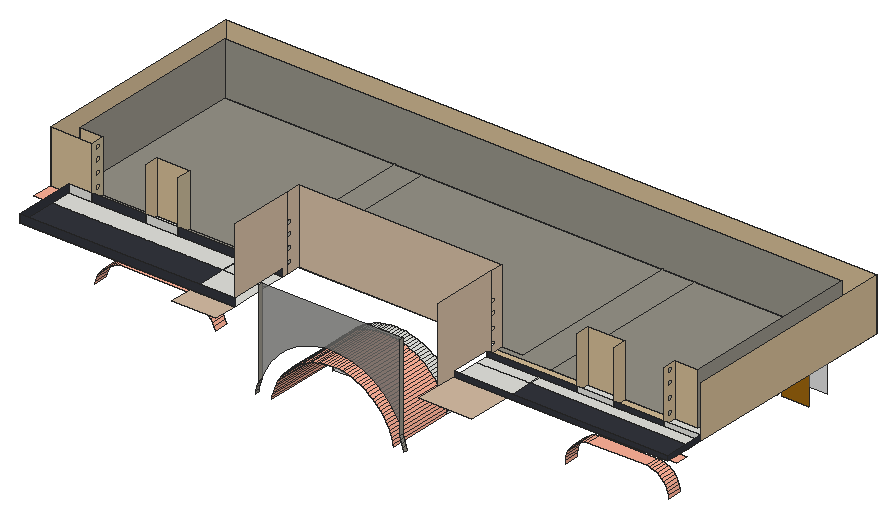
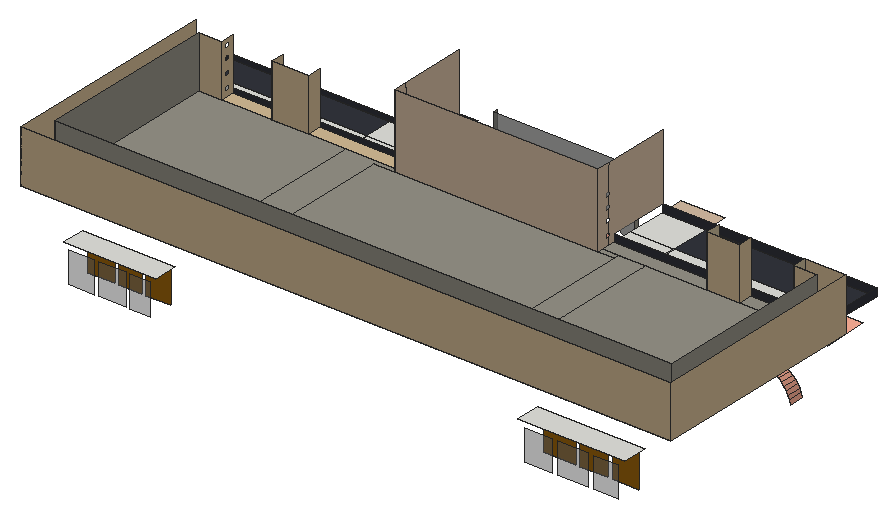
# SketchUp Ruby script. Lengths in inches.
U = 1.inch
M = Sketchup.active_model
def pt(a) = Geom::Point3d.new(a.map { |v| v * U })
def face(e, loops, mat)
  f = e.add_face(loops[0].map { |a| pt(a) })
  loops[1..].each { |l| e.add_face(l.map { |a| pt(a) }).erase! }
  f.material = f.back_material = mat if mat
  f
end
# faces: each face lists its corners as indices into pts; further lists are holes
def faces(e, pts, list, mat = nil) = list.each { |f| face(e, (f[0].is_a?(Array) ? f : [f]).map { |l| l.map { |i| pts[i] } }, mat) }
# xy, xz, yz: faces in a plane at the given z, y or x. An outline is a flat list of corners, or four numbers for a rectangle; further outlines are holes
def ring(l) = l.size == 4 ? [[l[0], l[1]], [l[2], l[1]], [l[2], l[3]], [l[0], l[3]]] : l.each_slice(2).to_a
def flat(e, list, mat, &to3) = list.each { |f| face(e, (f[0].is_a?(Array) ? f : [f]).map { |l| ring(l).map { |u, v| to3.(u, v) } }, mat) }
def xy(e, z, list, mat = nil) = flat(e, list, mat) { |x, y| [x, y, z] }
def xz(e, y, list, mat = nil) = flat(e, list, mat) { |x, z| [x, y, z] }
def yz(e, x, list, mat = nil) = flat(e, list, mat) { |y, z| [x, y, z] }
def lines(e, pts, list) = list.each { |a, b| e.add_line(pt(pts[a]), pt(pts[b])) }
# prism: a flat outline (further loops are holes) pulled along v
def prism(e, loops, v, mat = nil)
  f = face(e, loops, mat); d = Geom::Vector3d.new(v.map { |x| x * U })
  f.pushpull(f.normal.samedirection?(d) ? d.length : -d.length)
end
def box(e, o, s, mat = nil) = prism(e, [[o, [o[0] + s[0], o[1], o[2]], [o[0] + s[0], o[1] + s[1], o[2]], [o[0], o[1] + s[1], o[2]]]], [0, 0, s[2]], mat)
def at(x, y, z, deg = 0) = Geom::Transformation.translation(pt([x, y, z])) * Geom::Transformation.rotation(ORIGIN, Z_AXIS, deg.degrees)
def axes(o, x, y, z) = Geom::Transformation.new([*x, 0, *y, 0, *z, 0, *pt(o).to_a, 1])
def part(name) = M.definitions.add(name)
# library, detail: a bought-in or finely detailed component or shape, given as its bounding box
def library(name, o, s) = part(name).tap { |d| box(d.entities, o, s) }
def detail(e, o, s) = box(e.add_group.entities, o, s)
def put(e, d, t, mat = nil) = e.add_instance(d, t).tap { |i| i.material = mat if mat }
def group(e, t, mat = nil) = e.add_group.tap { |g| g.transformation = t; g.material = mat if mat }.entities
root = M.entities
M.materials.add("[Blinds Wood Light]").color = [155, 100, 14]
M.materials.add("[Color B02]").color = [255, 178, 153]
M.materials.add("[Formica Beige]").color = [211, 187, 149]
M.materials.add("[Formica Graystone]").color = [149, 146, 135]
M.materials.add("[Formica Laminate Dark]").color = [50, 53, 60]
M.materials.add("[Formica Laminate Light]").color = [213, 189, 164]
M.materials.add("[Quartz Light Brown]").color = [199, 184, 152]
M.materials.add("[Translucent Glass Block Dark]").color = [124, 124, 121]
M.materials["[Translucent Glass Block Dark]"].alpha = 0.8
M.materials.add("[Translucent Glass Gray]").color = [128, 128, 128]
M.materials["[Translucent Glass Gray]"].alpha = 0.5
M.materials.add("[Wood Veneer 01]3").color = [84, 49, 25]
xy(root,232.71,[[59.64,451.42,100.125,459.89]],"[Color B02]")
xy(root,236.125,[[341.29,451.42,376.4,459.89]],"[Color B02]")
xy(root,239.54,[[327.9375,568.57,383.25,583.14]])
xy(root,240.46,[[45.27,568.57,109.65,583.14]])
xy(root,249.06,[[311.91,444.11,400.54,451.42]],"[Color B02]")
xy(root,250.57,[[28.78,438.8,131.42,451.42]],"[Color B02]")
xy(root,261,[[131.42,414.84,157.59,438.8],[280.13,426.61,311.91,444.11],[28.78,438.8,131.42,451.42],[131.42,438.8,157.59,451.42],[280.13,444.11,311.91,451.42],
  [311.91,444.11,409.38,451.42],[17.625,451.42,17.625,583.14,409.38,583.14,409.38,451.42,386.6,451.42,386.6,459.89,400.54,459.89,400.54,568.57,28.78,568.57,28.78,459.89,42.4,459.89,42.4,451.42],[74.87,451.42,94.58,459.89],[334.34,451.42,356.76,459.89]])
xy(root,261,[[17.625,438.8,28.78,451.42]],"[Color B02]")
xy(root,261,[[280.13,451.42,334.34,459.89],[356.76,451.42,386.6,459.89]],"[Formica Beige]")
xy(root,261,[[42.4,451.42,74.87,459.89],[94.58,451.42,157.59,459.89],[28.78,459.89,131.42,568.57],[131.42,459.89,147.71,568.57],[147.71,459.89,157.59,463.02],
  [280.13,459.89,311.91,459.89,311.91,568.57,292.81,568.57,292.81,463.02,280.13,463.02],[311.91,459.89,400.54,568.57],[147.71,463.02,292.81,568.57]],"[Formica Graystone]")
xy(root,261,[[28.78,414.84,131.42,438.8],[311.91,426.61,409.38,444.11]],"[Formica Laminate Dark]")
xy(root,261,[[131.42,400.56,157.59,414.84],[280.13,400.56,311.91,426.61]],"[Formica Laminate Light]")
xz(root,414.84,[[28.78,261,157.59,265.6875]],"[Formica Laminate Dark]")
xz(root,414.84,[[174.14,227.22,174.4,227.97,175.18,229.93,176.05,231.85,177.02,233.73,178.07,235.57,179.2,237.35,180.42,239.08,181.71,240.75,183.08,242.36,184.53,243.9,186.04,245.375,187.63,246.77,189.27,248.1,190.98,249.34,192.74,250.51,194.56,251.59,196.42,252.59,198.33,253.49,200.28,254.3125,202.27,255.04,204.28,255.67,206.33,256.21,208.39,256.65,210.48,256.99,212.58,257.24,214.6875,257.39,216.8,257.44,218.91,257.39,221.02,257.24,223.12,256.99,225.21,256.65,227.27,256.21,229.32,255.67,231.33,255.04,233.32,254.3125,235.27,253.49,237.18,252.59,239.04,251.59,240.86,250.51,242.62,249.34,244.33,248.1,245.97,246.77,247.56,245.375,249.07,243.9,250.52,242.36,251.89,240.75,253.18,239.08,254.4,237.35,255.53,235.57,256.58,233.73,257.55,231.85,258.42,229.93,259.2,227.97,259.2,279.69,174.14,279.69]],"[Translucent Glass Block Dark]")
xz(root,426.61,[[280.13,261,409.38,263.9375]],"[Formica Laminate Dark]")
xz(root,451.42,[[28.78,261,42.4,265.6875],[74.87,261,94.58,265.6875],[334.34,261,356.76,263.9375],[386.6,261,409.38,263.9375]])
xz(root,451.42,[[17.625,261,28.78,261,28.78,265.6875,42.4,265.6875,42.4,292.375,17.625,292.375]],"[Formica Beige]")
xz(root,451.42,[[42.4,261,74.87,265.6875],[94.58,261,157.59,265.6875],[280.13,261,334.34,263.9375],[356.76,261,386.6,263.9375]],"[Formica Laminate Dark]")
xz(root,454.92,[[185.03,218.57,185.14,219.14,185.03,219.14],[248.46,218.57,248.57,218.57,248.46,219.14]])
xz(root,454.92,[[185.03,218.57,199.57,218.57,199.57,239.64,198.3,238.81,197.08,237.91,195.9,236.97,194.77,235.96,193.68,234.91,192.65,233.8,191.66,232.65,190.74,231.46,189.86,230.22,189.05,228.9375,188.3,227.625,187.61,226.28,186.99,224.9,186.42,223.49,185.93,222.0625,185.5,220.61,185.14,219.14],[202.18,218.57,213.78,218.57,213.78,244.46,212.27,244.29,210.78,244.04,209.3,243.72,207.83,243.34,206.39,242.89,204.97,242.37,203.57,241.78,202.2,241.13],[218.3125,218.57,233.875,218.57,234.03,239.64,232.73,240.42,231.4,241.13,230.03,241.78,228.63,242.37,227.21,242.89,225.77,243.34,224.3,243.72,222.82,244.04,221.33,244.29,219.82,244.46,218.3125,244.57],[236.52,218.57,248.46,218.57,248.46,219.14,248.1,220.61,247.67,222.0625,247.17,223.49,246.61,224.9,245.99,226.28,245.3,227.625,244.55,228.9375,243.73,230.22,242.86,231.46,241.9375,232.65,240.95,233.8,239.92,234.91,238.83,235.96,237.7,236.97,236.52,237.91]],"[Translucent Glass Gray]")
xz(root,454.92,[[199.57,218.57,202.18,218.57,202.2,241.13,200.87,240.42,199.57,239.64],[213.78,218.57,218.3125,218.57,218.3125,244.57,216.8,244.6,215.29,244.57,213.78,244.46],[233.875,218.57,236.52,218.57,236.52,237.91,235.3,238.81,234.03,239.64]],"[Wood Veneer 01]3")
xz(root,459.89,[[28.78,261,42.4,292.375],[74.87,261,94.58,292.375],[334.34,261,356.76,292.375],[386.6,261,400.54,292.375]],"[Formica Beige]")
xz(root,463.02,[[157.59,261,280.13,305.4375]],"[Formica Laminate Light]")
xz(root,568.57,[[48.75,217.42,64.6,236.99],[67.24,217.42,84.0625,236.99],[86.71,217.42,106.17,236.99],[330.49,217.74,345.72,236.98],[348.05,217.74,362.04,236.98],
  [364.37,217.74,380.69,236.98]],"[Blinds Wood Light]")
xz(root,568.57,[[28.78,261,400.54,292.375]],"[Formica Graystone]")
xz(root,583.14,[[17.625,261,409.38,292.375]],"[Formica Beige]")
xz(root,583.14,[[330.83,217.46,343.23,236.65],[345.56,217.46,362.04,236.65],[364.37,217.46,380.36,236.65],[49,218.21,64.12,236.74],[67.33,218.21,85.93,236.74],
  [89.14,218.21,105.92,236.74]],"[Translucent Glass Gray]")
yz(root,17.625,[[451.42,261,583.14,292.375]],"[Formica Beige]")
yz(root,28.78,[[459.89,261,568.57,292.375]],"[Formica Graystone]")
yz(root,28.78,[[414.84,261,451.42,265.6875]],"[Formica Laminate Dark]")
yz(root,42.4,[[[451.42,261,459.89,292.375],[456.03,265.2,455.63,265.25,455.25,265.41,454.93,265.66,454.68,265.98,454.52,266.36,454.47,266.76,454.52,267.17,454.68,267.54,454.93,267.87,455.25,268.11,455.63,268.27,456.03,268.32,456.4375,268.27,456.8125,268.11,457.14,267.87,457.39,267.54,457.54,267.17,457.6,266.76,457.54,266.36,457.39,265.98,457.14,265.66,456.8125,265.41,456.4375,265.25],[456.03,280.26,455.63,280.3125,455.25,280.47,454.93,280.72,454.68,281.04,454.52,281.42,454.47,281.82,454.52,282.23,454.68,282.6,454.93,282.93,455.25,283.18,455.63,283.33,456.03,283.39,456.4375,283.33,456.8125,283.18,457.14,282.93,457.39,282.6,457.54,282.23,457.6,281.82,457.54,281.42,457.39,281.04,457.14,280.72,456.8125,280.47,456.4375,280.3125],[456.03,273.07,455.63,273.125,455.25,273.28,454.93,273.53,454.68,273.85,454.52,274.23,454.47,274.64,454.52,275.04,454.68,275.42,454.93,275.74,455.25,275.99,455.63,276.15,456.03,276.2,456.4375,276.15,456.8125,275.99,457.14,275.74,457.39,275.42,457.54,275.04,457.6,274.64,457.54,274.23,457.39,273.85,457.14,273.53,456.8125,273.28,456.4375,273.125],[456.03,287.07,455.63,287.125,455.25,287.28,454.93,287.53,454.68,287.85,454.52,288.23,454.47,288.64,454.52,289.04,454.68,289.42,454.93,289.74,455.25,289.99,455.63,290.15,456.03,290.2,456.4375,290.15,456.8125,289.99,457.14,289.74,457.39,289.42,457.54,289.04,457.6,288.64,457.54,288.23,457.39,287.85,457.14,287.53,456.8125,287.28,456.4375,287.125]]],"[Quartz Light Brown]")
yz(root,74.87,[[451.42,261,459.89,292.375]],"[Formica Beige]")
yz(root,94.58,[[451.42,261,459.89,292.375]],"[Quartz Light Brown]")
yz(root,131.42,[[438.8,250.57,451.42,261]])
yz(root,157.59,[[451.42,261,451.42,265.6875,414.84,265.6875,414.84,305.4375,454.92,305.4375,454.92,289.73,454.68,289.42,454.52,289.04,454.47,288.64,454.52,288.23,454.68,287.85,454.92,287.54,454.92,282.92,454.68,282.6,454.52,282.23,454.47,281.82,454.52,281.42,454.68,281.04,454.92,280.73,454.92,275.73,454.68,275.42,454.52,275.04,454.47,274.64,454.52,274.23,454.68,273.85,454.92,273.54,454.92,267.86,454.68,267.54,454.52,267.17,454.47,266.76,454.52,266.36,454.68,265.98,454.92,265.66,454.92,261],[454.92,261,454.92,265.66,454.93,265.66,455.25,265.41,455.63,265.25,456.03,265.2,456.4375,265.25,456.8125,265.41,457.14,265.66,457.39,265.98,457.54,266.36,457.6,266.76,457.54,267.17,457.39,267.54,457.14,267.87,456.8125,268.11,456.4375,268.27,456.03,268.32,455.63,268.27,455.25,268.11,454.93,267.87,454.92,267.86,454.92,273.54,454.93,273.53,455.25,273.28,455.63,273.125,456.03,273.07,456.4375,273.125,456.8125,273.28,457.14,273.53,457.39,273.85,457.54,274.23,457.6,274.64,457.54,275.04,457.39,275.42,457.14,275.74,456.8125,275.99,456.4375,276.15,456.03,276.2,455.63,276.15,455.25,275.99,454.93,275.74,454.92,275.73,454.92,280.73,454.93,280.72,455.25,280.47,455.63,280.3125,456.03,280.26,456.4375,280.3125,456.8125,280.47,457.14,280.72,457.39,281.04,457.54,281.42,457.6,281.82,457.54,282.23,457.39,282.6,457.14,282.93,456.8125,283.18,456.4375,283.33,456.03,283.39,455.63,283.33,455.25,283.18,454.93,282.93,454.92,282.92,454.92,287.54,454.93,287.53,455.25,287.28,455.63,287.125,456.03,287.07,456.4375,287.125,456.8125,287.28,457.14,287.53,457.39,287.85,457.54,288.23,457.6,288.64,457.54,289.04,457.39,289.42,457.14,289.74,456.8125,289.99,456.4375,290.15,456.03,290.2,455.63,290.15,455.25,289.99,454.93,289.74,454.92,289.73,454.92,305.4375,463.02,305.4375,463.02,261]],"[Formica Laminate Light]")
yz(root,174.14,[[412.53,227.22,414.84,227.97],[412.53,227.97,414.84,279.69]],"[Formica Graystone]")
yz(root,259.2,[[412.53,227.97,414.84,279.69]],"[Formica Graystone]")
yz(root,280.13,[[414.84,261,426.61,261,426.61,263.9375,451.42,263.9375,451.42,261,454.92,261,454.92,264.8,454.76,265.01,454.61,265.38,454.55,265.79,454.61,266.19,454.76,266.57,454.92,266.78,454.92,272.86,454.76,273.07,454.61,273.45,454.55,273.85,454.61,274.26,454.76,274.63,454.92,274.84,454.92,281.24,454.76,281.44,454.61,281.82,454.55,282.23,454.61,282.63,454.76,283.01,454.92,283.21,454.92,287.99,454.76,288.19,454.61,288.57,454.55,288.98,454.61,289.38,454.76,289.76,454.92,289.96,454.92,305.4375,414.84,305.4375],[454.92,261,463.02,261,463.02,305.4375,454.92,305.4375,454.92,289.96,455.01,290.08,455.33,290.33,455.71,290.49,456.12,290.54,456.52,290.49,456.9,290.33,457.22,290.08,457.47,289.76,457.625,289.38,457.68,288.98,457.625,288.57,457.47,288.19,457.22,287.87,456.9,287.62,456.52,287.47,456.12,287.41,455.71,287.47,455.33,287.62,455.01,287.87,454.92,287.99,454.92,283.21,455.01,283.33,455.33,283.58,455.71,283.74,456.12,283.79,456.52,283.74,456.9,283.58,457.22,283.33,457.47,283.01,457.625,282.63,457.68,282.23,457.625,281.82,457.47,281.44,457.22,281.12,456.9,280.87,456.52,280.72,456.12,280.66,455.71,280.72,455.33,280.87,455.01,281.12,454.92,281.24,454.92,274.84,455.01,274.96,455.33,275.2,455.71,275.36,456.12,275.41,456.52,275.36,456.9,275.2,457.22,274.96,457.47,274.63,457.625,274.26,457.68,273.85,457.625,273.45,457.47,273.07,457.22,272.75,456.9,272.5,456.52,272.34,456.12,272.29,455.71,272.34,455.33,272.5,455.01,272.75,454.92,272.86,454.92,266.78,455.01,266.89,455.33,267.14,455.71,267.3,456.12,267.35,456.52,267.3,456.9,267.14,457.22,266.89,457.47,266.57,457.625,266.19,457.68,265.79,457.625,265.38,457.47,265.01,457.22,264.68,456.9,264.44,456.52,264.28,456.12,264.23,455.71,264.28,455.33,264.44,455.01,264.68,454.92,264.8]],"[Formica Laminate Light]")
yz(root,311.91,[[444.11,249.06,451.42,261]])
yz(root,334.34,[[451.42,261,459.89,292.375]],"[Formica Beige]")
yz(root,356.76,[[451.42,261,459.89,292.375]],"[Formica Beige]")
yz(root,386.6,[[[451.42,261,459.89,292.375],[456.12,287.41,456.52,287.47,456.9,287.62,457.22,287.87,457.47,288.19,457.625,288.57,457.68,288.98,457.625,289.38,457.47,289.76,457.22,290.08,456.9,290.33,456.52,290.49,456.12,290.54,455.71,290.49,455.33,290.33,455.01,290.08,454.76,289.76,454.61,289.38,454.55,288.98,454.61,288.57,454.76,288.19,455.01,287.87,455.33,287.62,455.71,287.47],[456.12,264.23,456.52,264.28,456.9,264.44,457.22,264.68,457.47,265.01,457.625,265.38,457.68,265.79,457.625,266.19,457.47,266.57,457.22,266.89,456.9,267.14,456.52,267.3,456.12,267.35,455.71,267.3,455.33,267.14,455.01,266.89,454.76,266.57,454.61,266.19,454.55,265.79,454.61,265.38,454.76,265.01,455.01,264.68,455.33,264.44,455.71,264.28],[456.12,280.66,456.52,280.72,456.9,280.87,457.22,281.12,457.47,281.44,457.625,281.82,457.68,282.23,457.625,282.63,457.47,283.01,457.22,283.33,456.9,283.58,456.52,283.74,456.12,283.79,455.71,283.74,455.33,283.58,455.01,283.33,454.76,283.01,454.61,282.63,454.55,282.23,454.61,281.82,454.76,281.44,455.01,281.12,455.33,280.87,455.71,280.72],[456.12,272.29,456.52,272.34,456.9,272.5,457.22,272.75,457.47,273.07,457.625,273.45,457.68,273.85,457.625,274.26,457.47,274.63,457.22,274.96,456.9,275.2,456.52,275.36,456.12,275.41,455.71,275.36,455.33,275.2,455.01,274.96,454.76,274.63,454.61,274.26,454.55,273.85,454.61,273.45,454.76,273.07,455.01,272.75,455.33,272.5,455.71,272.34]]],"[Formica Beige]")
yz(root,400.54,[[459.89,261,568.57,292.375]],"[Formica Graystone]")
yz(root,409.38,[[451.42,261,583.14,292.375]],"[Formica Beige]")
yz(root,409.38,[[426.61,261,451.42,263.9375]],"[Formica Laminate Dark]")
p = [[44.84,451.42,219.3],[44.2,451.42,217.08],[44.2,459.89,217.08],[44.84,459.89,219.3],[116.91,451.42,217.36],[116.1,451.42,219.36],
  [116.1,459.89,219.36],[116.91,459.89,217.36],[180.21,454.92,219.04],[180.43,454.92,220.17],[180.43,414.84,220.17],[180.21,414.84,219.04],
  [253.17,454.92,220.17],[253.39,454.92,219.04],[253.39,414.84,219.04],[253.17,414.84,220.17],[180.21,463.02,219.04],[180.43,463.02,220.17],
  [253.17,463.02,220.17],[253.39,463.02,219.04],[45.72,451.42,221.44],[45.72,459.89,221.44],[115.12,451.42,221.27],[115.12,459.89,221.27],
  [172.21,414.84,219.8125],[172.61,414.84,221.89],[172.61,412.53,221.89],[172.21,412.53,219.8125],[260.99,414.84,221.89],[261.39,414.84,219.8125],
  [261.39,412.53,219.8125],[260.99,412.53,221.89],[327.69,451.42,221.79],[327.58,451.42,219.87],[327.58,459.89,219.87],[327.69,459.89,221.79],
  [180.84,454.92,221.86],[180.84,414.84,221.86],[252.76,454.92,221.86],[252.76,414.84,221.86],[180.84,463.02,221.86],[252.76,463.02,221.86],
  [113.98,451.42,223.1],[113.98,459.89,223.1],[46.83,451.42,223.47],[46.83,459.89,223.47],[328.03,451.42,223.69],[328.03,459.89,223.69],
  [173.11,414.84,223.94],[173.11,412.53,223.94],[260.49,414.84,223.94],[260.49,412.53,223.94],[181.34,454.92,223.53],[181.34,414.84,223.53],
  [252.26,454.92,223.53],[252.26,414.84,223.53],[181.34,463.02,223.53],[252.26,463.02,223.53],[389.71,451.42,222.82],[389.59,451.42,224.56],
  [389.59,459.89,224.56],[389.71,459.89,222.82],[112.67,451.42,224.81],[112.67,459.89,224.81],[181.9,454.92,225.17],[181.9,414.84,225.17],
  [251.7,454.92,225.17],[251.7,414.84,225.17],[48.16,451.42,225.36],[48.16,459.89,225.36],[181.9,463.02,225.17],[251.7,463.02,225.17],
  [328.58,451.42,225.53],[328.58,459.89,225.53],[173.71,414.84,225.97],[173.71,412.53,225.97],[259.89,414.84,225.97],[259.89,412.53,225.97],
  [389.25,451.42,226.26],[389.25,459.89,226.26],[111.22,451.42,226.4],[111.22,459.89,226.4],[182.55,454.92,226.79],[182.55,414.84,226.79],
  [251.05,454.92,226.79],[251.05,414.84,226.79],[182.55,463.02,226.79],[251.05,463.02,226.79],[49.6875,451.42,227.1],[49.6875,459.89,227.1],
  [329.35,451.42,227.29],[329.35,459.89,227.29],[174.14,414.84,227.22],[174.14,412.53,227.22],[259.2,414.84,227.97],[259.2,412.53,227.97],
  [388.69,451.42,227.91],[388.69,459.89,227.91],[109.63,451.42,227.85],[109.63,459.89,227.85],[183.27,454.92,228.375],[183.27,414.84,228.375],
  [250.33,454.92,228.375],[250.33,414.84,228.375],[183.27,463.02,228.375],[250.33,463.02,228.375],[51.4,451.42,228.65],[51.4,459.89,228.65],
  [330.3125,451.42,228.96],[330.3125,459.89,228.96],[107.92,451.42,229.15],[107.92,459.89,229.15],[387.92,451.42,229.47],[387.92,459.89,229.47],
  [184.06,454.92,229.92],[184.06,414.84,229.92],[249.54,454.92,229.92],[249.54,414.84,229.92],[184.06,463.02,229.92],[249.54,463.02,229.92],
  [53.28,451.42,230],[53.28,459.89,230],[331.47,451.42,230.5],[331.47,459.89,230.5],[106.1,451.42,230.3],[106.1,459.89,230.3],
  [386.96,451.42,230.92],[386.96,459.89,230.92],[184.92,454.92,231.43],[184.92,414.84,231.43],[248.68,454.92,231.43],[248.68,414.84,231.43],
  [184.92,463.02,231.43],[248.68,463.02,231.43],[55.3,451.42,231.14],[55.3,459.89,231.14],[104.18,451.42,231.28],[104.18,459.89,231.28],
  [332.79,451.42,231.9],[332.79,459.89,231.9],[385.81,451.42,232.23],[385.81,459.89,232.23],[57.43,451.42,232.04],[57.43,459.89,232.04],
  [102.18,451.42,232.08],[102.18,459.89,232.08],[185.86,454.92,232.9],[185.86,414.84,232.9],[247.74,454.92,232.9],[247.74,414.84,232.9],
  [185.86,463.02,232.9],[247.74,463.02,232.9],[334.27,451.42,233.13],[334.27,459.89,233.13],[59.64,451.42,232.71],[59.64,459.89,232.71],
  [100.125,451.42,232.71],[100.125,459.89,232.71],[384.5,451.42,233.375],[384.5,459.89,233.375],[186.86,454.92,234.32],[186.86,414.84,234.32],
  [246.74,454.92,234.32],[246.74,414.84,234.32],[186.86,463.02,234.32],[246.74,463.02,234.32],[335.88,451.42,234.18],[335.88,459.89,234.18],
  [383.05,451.42,234.34],[383.05,459.89,234.34],[337.6,451.42,235.04],[337.6,459.89,235.04],[187.92,454.92,235.7],[187.92,414.84,235.7],
  [245.68,454.92,235.7],[245.68,414.84,235.7],[381.49,451.42,235.11],[381.49,459.89,235.11],[187.92,463.02,235.7],[245.68,463.02,235.7],
  [339.41,451.42,235.6875],[339.41,459.89,235.6875],[379.85,451.42,235.67],[379.85,459.89,235.67],[189.05,454.92,237.02],[189.05,414.84,237.02],
  [244.55,454.92,237.02],[244.55,414.84,237.02],[341.29,451.42,236.125],[341.29,459.89,236.125],[378.14,451.42,236.01],[378.14,459.89,236.01],
  [189.05,463.02,237.02],[244.55,463.02,237.02],[376.4,451.42,236.125],[376.4,459.89,236.125],[190.24,454.92,238.29],[190.24,414.84,238.29],
  [243.36,454.92,238.29],[243.36,414.84,238.29],[190.24,463.02,238.29],[243.36,463.02,238.29],[191.49,454.92,239.5],[191.49,414.84,239.5],
  [242.11,454.92,239.5],[242.11,414.84,239.5],[191.49,463.02,239.5],[242.11,463.02,239.5],[192.79,454.92,240.65],[192.79,414.84,240.65],
  [240.81,454.92,240.65],[240.81,414.84,240.65],[192.79,463.02,240.65],[240.81,463.02,240.65],[194.15,454.92,241.74],[194.15,414.84,241.74],
  [239.45,454.92,241.74],[239.45,414.84,241.74],[194.15,463.02,241.74],[239.45,463.02,241.74],[195.55,454.92,242.77],[195.55,414.84,242.77],
  [238.05,454.92,242.77],[238.05,414.84,242.77],[195.55,463.02,242.77],[238.05,463.02,242.77],[197,454.92,243.73],[197,414.84,243.73],
  [236.6,454.92,243.73],[236.6,414.84,243.73],[197,463.02,243.73],[236.6,463.02,243.73],[198.5,454.92,244.62],[198.5,414.84,244.62],
  [235.1,454.92,244.62],[235.1,414.84,244.62],[198.5,463.02,244.62],[235.1,463.02,244.62],[200.03,454.92,245.4375],[200.03,414.84,245.4375],
  [233.57,454.92,245.4375],[233.57,414.84,245.4375],[200.03,463.02,245.4375],[233.57,463.02,245.4375],[201.6,454.92,246.18],[201.6,414.84,246.18],
  [232,454.92,246.18],[232,414.84,246.18],[201.6,463.02,246.18],[232,463.02,246.18],[203.21,454.92,246.86],[203.21,414.84,246.86],
  [230.39,454.92,246.86],[230.39,414.84,246.86],[203.21,463.02,246.86],[230.39,463.02,246.86],[204.84,454.92,247.45],[204.84,414.84,247.45],
  [228.76,454.92,247.45],[228.76,414.84,247.45],[204.84,463.02,247.45],[228.76,463.02,247.45],[206.5,454.92,247.97],[206.5,414.84,247.97],
  [227.1,454.92,247.97],[227.1,414.84,247.97],[206.5,463.02,247.97],[227.1,463.02,247.97],[208.18,454.92,248.42],[208.18,414.84,248.42],
  [225.42,454.92,248.42],[225.42,414.84,248.42],[208.18,463.02,248.42],[225.42,463.02,248.42],[209.88,454.92,248.78],[209.88,414.84,248.78],
  [223.72,454.92,248.78],[223.72,414.84,248.78],[209.88,463.02,248.78],[223.72,463.02,248.78],[211.6,454.92,249.0625],[211.6,414.84,249.0625],
  [222,454.92,249.0625],[222,414.84,249.0625],[211.6,463.02,249.0625],[222,463.02,249.0625],[213.33,454.92,249.27],[213.33,414.84,249.27],
  [220.27,454.92,249.27],[220.27,414.84,249.27],[213.33,463.02,249.27],[220.27,463.02,249.27],[215.0625,454.92,249.39],[215.0625,414.84,249.39],
  [218.54,454.92,249.39],[218.54,414.84,249.39],[215.0625,463.02,249.39],[218.54,463.02,249.39],[216.8,454.92,249.43],[216.8,414.84,249.43],
  [216.8,463.02,249.43]]
faces(root,p,[[0,1,2,3],[4,5,6,7],[8,9,10,11],[12,13,14,15],[20,0,3,21],[5,22,23,6],[32,33,34,35],[9,36,37,10],
  [38,12,15,39],[22,42,43,23],[44,20,21,45],[46,32,35,47],[36,52,53,37],[54,38,39,55],[58,59,60,61],[42,62,63,43],
  [52,64,65,53],[66,54,55,67],[68,44,45,69],[72,46,47,73],[59,78,79,60],[62,80,81,63],[64,82,83,65],[84,66,67,85],
  [88,68,69,89],[90,72,73,91],[78,96,97,79],[80,98,99,81],[82,100,101,83],[102,84,85,103],[106,88,89,107],[108,90,91,109],
  [98,110,111,99],[96,112,113,97],[100,114,115,101],[116,102,103,117],[120,106,107,121],[122,108,109,123],[110,124,125,111],[112,126,127,113],
  [114,128,129,115],[130,116,117,131],[134,120,121,135],[124,136,137,125],[138,122,123,139],[126,140,141,127],[142,134,135,143],[136,144,145,137],
  [128,146,147,129],[148,130,131,149],[152,138,139,153],[154,142,143,155],[144,156,157,145],[140,158,159,141],[146,160,161,147],[162,148,149,163],
  [166,152,153,167],[158,168,169,159],[170,166,167,171],[160,172,173,161],[174,162,163,175],[168,176,177,169],[180,170,171,181],[176,182,183,177],
  [172,184,185,173],[186,174,175,187],[188,180,181,189],[182,190,191,183],[190,194,195,191],[184,196,197,185],[198,186,187,199],[196,202,203,197],
  [204,198,199,205],[202,208,209,203],[210,204,205,211],[208,214,215,209],[216,210,211,217],[214,220,221,215],[222,216,217,223],[220,226,227,221],
  [228,222,223,229],[226,232,233,227],[234,228,229,235],[232,238,239,233],[240,234,235,241],[238,244,245,239],[246,240,241,247],[244,250,251,245],
  [252,246,247,253],[250,256,257,251],[258,252,253,259],[256,262,263,257],[264,258,259,265],[262,268,269,263],[270,264,265,271],[268,274,275,269],
  [276,270,271,277],[274,280,281,275],[282,276,277,283],[280,286,287,281],[288,282,283,289],[286,292,293,287],[294,288,289,295],[292,298,299,293],
  [298,294,295,299]],"[Color B02]")
faces(root,p,[[9,8,16,17],[13,12,18,19],[36,9,17,40],[12,38,41,18],[52,36,40,56],[38,54,57,41],[64,52,56,70],[54,66,71,57],
  [82,64,70,86],[66,84,87,71],[100,82,86,104],[84,102,105,87],[114,100,104,118],[102,116,119,105],[128,114,118,132],[116,130,133,119],
  [146,128,132,150],[130,148,151,133],[160,146,150,164],[148,162,165,151],[172,160,164,178],[162,174,179,165],[184,172,178,192],[174,186,193,179],
  [196,184,192,200],[186,198,201,193],[202,196,200,206],[198,204,207,201],[208,202,206,212],[204,210,213,207],[214,208,212,218],[210,216,219,213],
  [220,214,218,224],[216,222,225,219],[226,220,224,230],[222,228,231,225],[232,226,230,236],[228,234,237,231],[238,232,236,242],[234,240,243,237],
  [244,238,242,248],[240,246,249,243],[250,244,248,254],[246,252,255,249],[256,250,254,260],[252,258,261,255],[262,256,260,266],[258,264,267,261],
  [268,262,266,272],[264,270,273,267],[274,268,272,278],[270,276,279,273],[280,274,278,284],[276,282,285,279],[286,280,284,290],[282,288,291,285],
  [292,286,290,296],[288,294,297,291],[298,292,296,300],[294,298,300,297]])
faces(root,p,[[24,25,26,27],[28,29,30,31],[25,48,49,26],[50,28,31,51],[48,74,75,49],[76,50,51,77],[74,92,93,75],[94,76,77,95]],"[Formica Graystone]")
